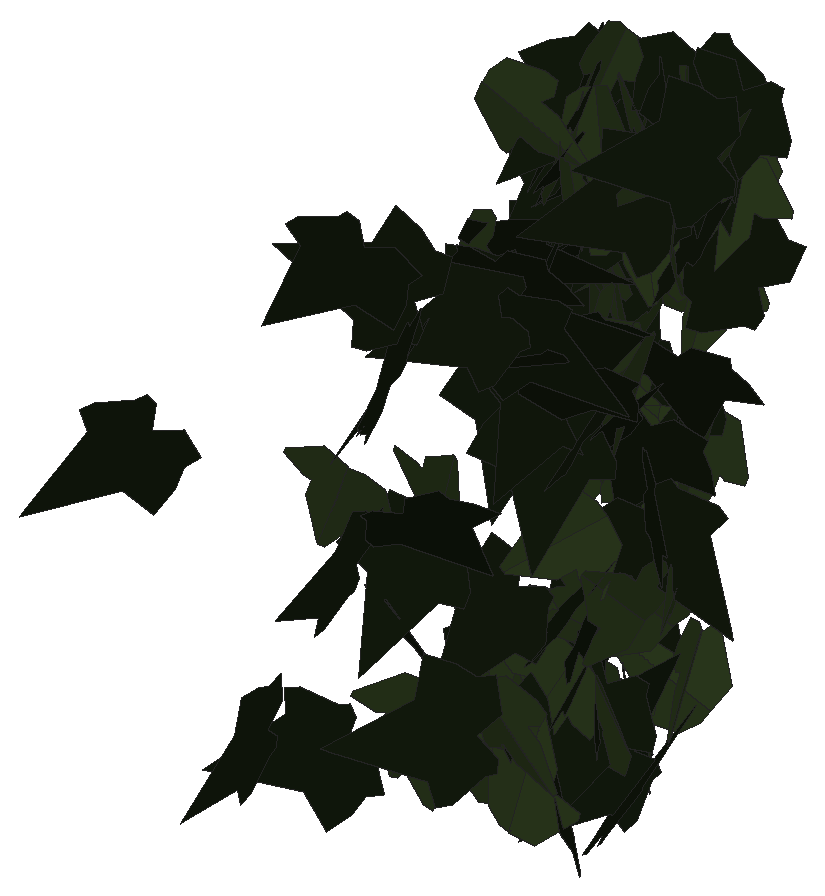
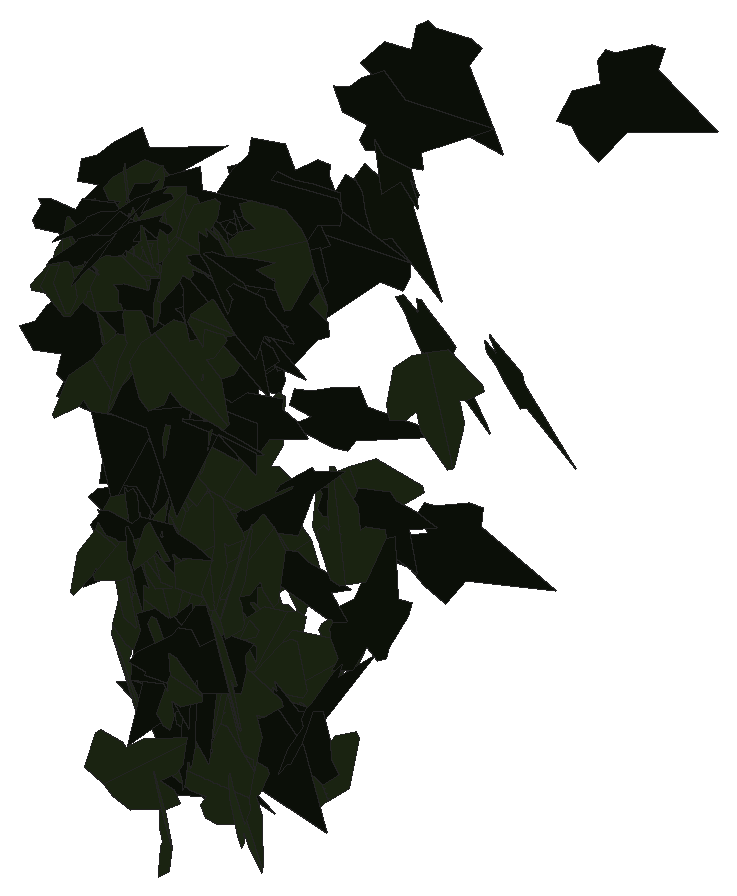
# SketchUp Ruby script. Lengths in inches.
U = 1.inch
M = Sketchup.active_model
def pt(a) = Geom::Point3d.new(a.map { |v| v * U })
def face(e, loops, mat)
  f = e.add_face(loops[0].map { |a| pt(a) })
  loops[1..].each { |l| e.add_face(l.map { |a| pt(a) }).erase! }
  f.material = f.back_material = mat if mat
  f
end
# faces: each face lists its corners as indices into pts; further lists are holes
def faces(e, pts, list, mat = nil) = list.each { |f| face(e, (f[0].is_a?(Array) ? f : [f]).map { |l| l.map { |i| pts[i] } }, mat) }
# xy, xz, yz: faces in a plane at the given z, y or x. An outline is a flat list of corners, or four numbers for a rectangle; further outlines are holes
def ring(l) = l.size == 4 ? [[l[0], l[1]], [l[2], l[1]], [l[2], l[3]], [l[0], l[3]]] : l.each_slice(2).to_a
def flat(e, list, mat, &to3) = list.each { |f| face(e, (f[0].is_a?(Array) ? f : [f]).map { |l| ring(l).map { |u, v| to3.(u, v) } }, mat) }
def xy(e, z, list, mat = nil) = flat(e, list, mat) { |x, y| [x, y, z] }
def xz(e, y, list, mat = nil) = flat(e, list, mat) { |x, z| [x, y, z] }
def yz(e, x, list, mat = nil) = flat(e, list, mat) { |y, z| [x, y, z] }
def lines(e, pts, list) = list.each { |a, b| e.add_line(pt(pts[a]), pt(pts[b])) }
# prism: a flat outline (further loops are holes) pulled along v
def prism(e, loops, v, mat = nil)
  f = face(e, loops, mat); d = Geom::Vector3d.new(v.map { |x| x * U })
  f.pushpull(f.normal.samedirection?(d) ? d.length : -d.length)
end
def box(e, o, s, mat = nil) = prism(e, [[o, [o[0] + s[0], o[1], o[2]], [o[0] + s[0], o[1] + s[1], o[2]], [o[0], o[1] + s[1], o[2]]]], [0, 0, s[2]], mat)
def at(x, y, z, deg = 0) = Geom::Transformation.translation(pt([x, y, z])) * Geom::Transformation.rotation(ORIGIN, Z_AXIS, deg.degrees)
def axes(o, x, y, z) = Geom::Transformation.new([*x, 0, *y, 0, *z, 0, *pt(o).to_a, 1])
def part(name) = M.definitions.add(name)
# library, detail: a bought-in or finely detailed component or shape, given as its bounding box
def library(name, o, s) = part(name).tap { |d| box(d.entities, o, s) }
def detail(e, o, s) = box(e.add_group.entities, o, s)
def put(e, d, t, mat = nil) = e.add_instance(d, t).tap { |i| i.material = mat if mat }
def group(e, t, mat = nil) = e.add_group.tap { |g| g.transformation = t; g.material = mat if mat }.entities
root = M.entities
M.materials.add("efeu1").color = [18, 25, 13]
M.materials.add("efeu2").color = [43, 57, 29]
c1 = part("ivyleaf_9")
p = [[1.54,2.16,1.25],[1.36,2.04,1.19],[-0.21,0.99,0.68],[-0.71,1.11,0.82],[-0.85,0.86,0.67],[-0.8,0.17,0.21],
  [-0.9,-0.01,0.1],[-0.67,-0.16,-0.02],[-0.08,-0.08,-0.05],[-0.03,-0.6,-0.4],[0.65,-0.88,-0.66],[0.83,-0.6,-0.49],
  [1.29,-0.42,-0.43],[1.8125,-0.07,-0.26],[1.21,0.44,0.15]]
faces(c1.entities,p,[[0,1,2,3,4,5,6,7,8,9,10,11,12,13,14]],"efeu1")
c2 = part("ivyleaf_10")
p = [[0,0.5,-0.03],[-0.0625,2.02,-0.43],[-0.19,2.01,-0.46],[-0.54,1.05,-0.29],[-0.52,0.625,-0.18],[-0.83,0.76,-0.28],
  [-1.16,0.64,-0.33],[-1.15,0.33,-0.24],[-0.77,-0.39,0.02],[-0.3,-0.51,0.16],[0.04,-0.48,0.23],[-0.02,2.01,-0.4375],
  [-0.06,2.01,-0.43],[0.04,-0.49,0.23],[0.67,-0.49,0.14],[1.38,0.36,-0.2],[1.375,0.51,-0.24],[0.81,0.65,-0.19],
  [0.62,0.59,-0.15],[0.6,1.09,-0.28],[0.5,1.23,-0.31]]
faces(c2.entities,p,[[0,1,2,3,4,5,6,7,8,9,10],[11,12,0,13,14,15,16,17,18,19,20]],"efeu2")
put(root,c1,axes([51.93,217.2,212.98],[-0.05869,0.02643,-0.49584],[-0.02771,-0.49869,-0.02331],[-0.49577,0.02474,0.06]))
put(root,c1,axes([52.75,217.98,209.62],[-0.43052,0.24134,-0.08007],[0.06799,-0.04247,-0.49353],[-0.24502,-0.43584,0.00375]))
put(root,c1,axes([53.94,219.7,209.25],[-0.36119,-0.02977,0.34447],[-0.33695,-0.08134,-0.36034],[0.0775,-0.49244,0.0387]))
put(root,c1,axes([52.6875,219.4375,210.8],[-0.36273,0.34249,0.03353],[-0.02659,0.02067,-0.49886],[-0.3431,-0.36369,0.00322]))
put(root,c1,axes([52.63,219.63,214.2],[0.07664,0.12487,-0.47805],[-0.2722,-0.39307,-0.14631],[-0.41235,0.28268,0.00773]))
put(root,c1,axes([53.43,219.36,211.66],[0.38543,0.31697,0.03117],[0.02393,0.01998,-0.49903],[-0.3176,0.38617,0.00023]))
put(root,c1,axes([52.1875,219.87,208.45],[-0.09347,-0.05912,-0.48761],[-0.29492,-0.39018,0.10384],[-0.39279,0.30703,0.03807]))
put(root,c1,axes([53.15,219.4375,213],[-0.26005,0.14295,-0.40242],[-0.35072,0.19733,0.29674],[0.24366,0.43661,-0.00237]))
put(root,c1,axes([52.75,220.04,212.73],[-0.3149,0.36073,-0.14391],[0.09485,-0.10823,-0.47884],[-0.37662,-0.32887,-0.00026]))
put(root,c1,axes([52.8,220.15,213.5],[-0.19213,0.03222,0.46049],[-0.45006,0.09779,-0.19462],[-0.10261,-0.48928,-0.00858]))
put(root,c2,axes([52.88,220.35,208.99],[-0.34204,-0.31812,0.17834],[-0.12668,-0.12564,-0.46708],[0.34199,-0.36471,0.00535]))
put(root,c2,axes([51.69,220.57,210.91],[-0.44087,-0.09357,0.21651],[-0.21259,-0.04117,-0.45068],[0.10217,-0.48944,-0.00348]))
put(root,c1,axes([53.06,221.26,212.93],[-0.44488,0.00063,0.22821],[-0.2282,0.0041,-0.44487],[-0.00243,-0.49998,-0.00336]))
put(root,c2,axes([53.04,221.24,208.59],[-0.34431,0.11872,-0.34257],[0.31834,-0.12712,-0.36401],[-0.17352,-0.46877,0.01195]))
put(root,c2,axes([53.32,221.22,207.57],[0.49184,-0.06443,-0.06276],[0.06362,0.00252,0.49593],[-0.06359,-0.49582,0.01068]))
put(root,c1,axes([53.13,221.28,212.82],[-0.00254,0.00286,-0.49999],[0.32697,0.37827,0.0005],[0.37827,-0.32696,-0.00379]))
put(root,c1,axes([51.81,221.65,209.79],[-0.43015,-0.23233,-0.10487],[0.09824,0.03872,-0.48872],[0.23521,-0.44105,0.01234]))
put(root,c1,axes([53.32,221.89,207.32],[0.01934,-0.13736,0.48037],[0.09828,-0.47029,-0.13844],[0.48986,0.09978,0.00881]))
put(root,c2,axes([52.15,221.25,207.87],[-0.05823,0.33651,0.3652],[-0.08192,0.35616,-0.34124],[-0.48979,-0.09957,0.01365]))
put(root,c1,axes([52.92,221.4,213.36],[0.37757,0.25861,-0.2014],[-0.16846,-0.11045,-0.45763],[-0.28118,0.41343,0.00373]))
put(root,c1,axes([53.12,221.95,211.875],[-0.13061,-0.44021,0.19788],[-0.03696,-0.19528,-0.4588],[0.48122,-0.13448,0.01847]))
put(root,c1,axes([53.29,221.82,211.52],[-0.196,-0.45231,-0.08365],[0.02284,0.08124,-0.49283],[0.45941,-0.19701,-0.01119]))
put(root,c1,axes([53.73,221.59,212.36],[0.10603,0.32943,-0.36088],[-0.27049,-0.26797,-0.32408],[-0.40693,0.26395,0.12139]))
put(root,c1,axes([51.4,221.99,208.34],[0.42363,-0.26443,-0.02474],[0.03192,0.00445,0.49896],[-0.26366,-0.42433,0.02065]))
put(root,c1,axes([53.04,222.08,212.15],[0.02976,-0.02806,0.49832],[0.40241,-0.29397,-0.04059],[0.29527,0.40348,0.00508]))
put(root,c1,axes([53.57,221.85,211.4375],[-0.20148,0.4259,0.16738],[-0.10421,0.13538,-0.46991],[-0.44559,-0.22424,0.03421]))
put(root,c2,axes([51.84,222.36,212.6875],[-0.0193,-0.03197,-0.4986],[0.33338,-0.37248,0.01098],[-0.37214,-0.33202,0.03569]))
put(root,c1,axes([52.36,222.34,209.14],[-0.47848,-0.13346,-0.05695],[0.05755,0.0056,-0.49665],[0.1332,-0.48183,0.01]))
put(root,c2,axes([51.3,222.49,209.61],[-0.43722,0.08105,0.22863],[0.22455,-0.04302,0.44467],[0.09175,0.49151,0.00123]))
put(root,c1,axes([51.55,222.87,207.64],[0.14864,-0.28493,-0.38304],[0.22933,-0.30924,0.31902],[-0.41871,-0.27053,0.03876]))
put(root,c2,axes([52.8125,222.51,208.34],[0.45497,-0.06468,-0.19703],[-0.19487,0.0291,-0.45954],[0.07091,0.49494,0.00128]))
put(root,c1,axes([52.34,222.53,212.04],[-0.03092,0.36078,0.3448],[0.01889,-0.34436,0.36202],[0.49869,0.03542,0.00767]))
put(root,c2,axes([51.55,222.59,206.85],[-0.38038,-0.0109,0.32433],[0.32434,0.00379,0.38051],[-0.01075,0.49987,0.00419]))
put(root,c2,axes([51.94,222.21,207.86],[0.0691,0.11293,0.48215],[0.08248,0.4774,-0.12363],[-0.48829,0.09662,0.04734]))
put(root,c2,axes([52.95,222.68,209.9],[0.32792,0.01853,-0.377],[-0.37564,-0.03294,-0.32835],[-0.037,0.49857,-0.00768]))
put(root,c1,axes([53.07,222.39,209.17],[-0.17356,0.45442,0.11566],[-0.06062,0.10055,-0.48602],[-0.46498,-0.18273,0.02019]))
put(root,c1,axes([53.4,222.24,211.17],[0.10808,0.41603,0.25542],[0.02456,0.25664,-0.42841],[-0.48756,0.10515,0.03504]))
put(root,c1,axes([52.91,222.76,208.43],[-0.36094,0.22076,-0.26643],[0.21911,-0.15213,-0.4229],[-0.26778,-0.42204,0.01308]))
put(root,c1,axes([52.98,222.96,208],[-0.24907,-0.4328,0.02543],[0.01012,-0.03513,-0.49866],[0.43343,-0.24788,0.02626]))
put(root,c2,axes([53.52,222.47,207.88],[-0.14103,0.1618,-0.45159],[-0.32263,0.31634,0.2141],[0.35499,0.35178,0.01518]))
put(root,c1,axes([51.7,222.76,207.06],[-0.14899,0.10833,0.46483],[0.32585,-0.33272,0.18198],[0.34874,0.35716,0.02854]))
put(root,c2,axes([53.14,223.1,211.6],[-0.00318,-0.08574,0.49258],[0.13006,-0.47578,-0.08197],[0.48278,0.12761,0.02533]))
put(root,c2,axes([53.3125,223.04,208.92],[-0.12369,-0.31974,-0.36396],[-0.14542,-0.33381,0.34267],[-0.46212,0.19063,-0.01042]))
put(root,c1,axes([51.87,222.54,212.63],[0.37549,0.06671,0.32335],[0.31648,0.06677,-0.38129],[-0.09405,0.49101,0.00792]))
put(root,c1,axes([53.41,222.49,206.82],[-0.19352,0.45369,-0.08194],[-0.03315,0.07495,0.49324],[0.45984,0.19633,0.00108]))
put(root,c1,axes([52.7,222.59,211.97],[0.33303,0.3726,-0.01596],[-0.01069,-0.01185,-0.49975],[-0.37279,0.33321,0.00007]))
put(root,c1,axes([52.32,222.85,207.35],[0.02988,0.23247,-0.44166],[-0.37496,-0.28157,-0.17357],[-0.32942,0.34158,0.1575]))
put(root,c2,axes([52.15,222.67,208.53],[0.09058,0.43775,0.22398],[0.02329,0.22367,-0.44657],[-0.49117,0.09134,0.02013]))
put(root,c1,axes([53.49,223.2,213.49],[-0.2892,-0.17302,0.36936],[-0.32093,-0.18292,-0.33697],[0.25173,-0.43198,-0.00525]))
put(root,c2,axes([52.75,223.1875,211.74],[0.07905,-0.10737,-0.4819],[0.26888,-0.39995,0.13322],[-0.41407,-0.28021,-0.0055]))
put(root,c2,axes([53.3125,223.13,211.71],[0.22234,-0.40073,0.19996],[0.09517,-0.17586,-0.45827],[0.43761,0.24185,-0.00193]))
put(root,c2,axes([52.22,222.8,208.28],[-0.21629,-0.35255,-0.28094],[0.14733,0.23921,-0.41361],[0.42604,-0.2617,0.0004]))
put(root,c1,axes([52.91,222.82,208],[0.08149,-0.0056,-0.49328],[-0.48911,0.06421,-0.08153],[0.06426,0.49583,0.00499]))
put(root,c1,axes([53.07,223.23,207.19],[-0.49847,0.0167,0.03535],[-0.03569,-0.01007,-0.49862],[-0.01595,-0.49962,0.01123]))
put(root,c1,axes([52.95,222.9,207.4375],[-0.22353,0.43739,0.09344],[-0.04941,0.07967,-0.49113],[-0.44452,-0.2288,0.00761]))
put(root,c2,axes([52.8125,223.22,208.75],[-0.4478,-0.04873,-0.21704],[-0.21272,-0.0488,0.44985],[-0.06502,0.49522,0.02297]))
put(root,c1,axes([51.56,223.46,210.69],[-0.11731,-0.48455,0.03803],[-0.00547,-0.0378,-0.49854],[0.48601,-0.11738,0.00356]))
put(root,c1,axes([52.84,222.8125,208.25],[0.03725,0.03445,0.49742],[0.17231,0.46719,-0.04526],[-0.46789,0.17479,0.02294]))
put(root,c1,axes([53.81,223.58,213.92],[-0.21312,-0.12866,0.43362],[-0.34871,-0.25855,-0.2481],[0.28807,-0.40816,0.02047]))
put(root,c1,axes([53.43,223.1,210.26],[0.23797,-0.09851,-0.42856],[-0.39489,0.16652,-0.25755],[0.19347,0.46105,0.00145]))
put(root,c2,axes([52.35,223.31,207.93],[-0.43351,-0.13752,0.20775],[-0.19934,-0.05864,-0.45478],[0.14945,-0.47713,-0.00399]))
put(root,c1,axes([53.28,223.31,210.83],[0.25711,0.20304,-0.37771],[-0.28476,-0.24845,-0.32739],[-0.32064,0.38346,-0.01212]))
put(root,c2,axes([53.13,223.62,208.57],[-0.23156,-0.26907,-0.35211],[-0.2427,-0.2554,0.35478],[-0.37078,0.33522,-0.01232]))
put(root,c2,axes([51.45,223.36,213.87],[-0.24625,0.0433,-0.433],[0.42583,-0.07849,-0.25002],[-0.08962,-0.4919,0.00178]))
put(root,c1,axes([53.29,223.29,209.88],[-0.11782,-0.18414,-0.44968],[0.24248,0.37871,-0.2186],[0.4211,-0.26958,0.00006]))
put(root,c1,axes([52.46,223.21,206.98],[-0.04662,-0.14522,0.47617],[0.46851,0.14888,0.09128],[-0.16829,0.45469,0.12219]))
put(root,c2,axes([53.43,223.18,213.75],[-0.18692,-0.25812,-0.38527],[0.21897,0.31705,-0.31865],[0.4088,-0.28784,-0.00548]))
put(root,c2,axes([53.68,223.18,213.02],[-0.03548,0.02569,0.49808],[-0.41201,0.27987,-0.04378],[-0.28104,-0.41354,0.00131]))
put(root,c2,axes([53.3,223.82,209.26],[0.07977,-0.12907,0.47642],[0.29408,-0.37517,-0.15088],[0.39642,0.30429,0.01606]))
put(root,c2,axes([53.04,223.45,213.18],[0.29978,0.39559,0.06035],[0.03471,0.04941,-0.49634],[-0.39866,0.30177,0.00217]))
put(root,c2,axes([51.7,223.51,210.15],[-0.41829,0.14489,-0.23246],[0.2161,-0.08617,-0.44258],[-0.16832,-0.47072,0.00947]))
put(root,c2,axes([52.72,223.83,211.36],[0.02205,-0.32082,-0.38287],[0.11483,-0.36972,0.31642],[-0.48614,-0.10188,0.05737]))
put(root,c2,axes([52.29,223.64,213.84],[0.42049,-0.13497,0.23446],[0.2362,-0.02811,-0.43979],[0.1319,0.48062,0.04012]))
put(root,c2,axes([53.45,223.71,208.24],[0.31321,-0.38603,0.05366],[0.03384,-0.04164,-0.49711],[0.38827,0.31503,0.00005]))
put(root,c1,axes([53.53,223.45,211.62],[0.35215,0.26501,-0.23614],[-0.19765,-0.1299,-0.44052],[-0.29483,0.40361,0.01327]))
put(root,c1,axes([52.0625,223.86,213],[-0.47016,-0.1664,0.03554],[-0.02789,-0.02768,-0.49845],[0.16786,-0.47068,0.01675]))
put(root,c1,axes([53.76,223.29,212.92],[-0.32596,0.29399,-0.23942],[-0.17355,0.16502,0.43892],[0.33709,0.36924,-0.00554]))
put(root,c2,axes([52.05,223.625,213.32],[-0.15688,0.4703,-0.06488],[0.00927,-0.06528,-0.49563],[-0.47466,-0.15671,0.01176]))
put(root,c2,axes([53.19,223.53,213.5625],[-0.28541,0.23891,-0.33386],[-0.26779,0.19986,0.37194],[0.31117,0.39112,0.01387]))
put(root,c2,axes([51.73,223.91,211.13],[-0.25426,-0.30277,-0.30607],[-0.19788,-0.2335,0.39537],[-0.38235,0.32219,-0.00108]))
put(root,c2,axes([52.67,224,213.42],[-0.04976,0.146,-0.47561],[0.08246,-0.46895,-0.15258],[-0.49064,-0.09363,0.02259]))
put(root,c2,axes([51.73,223.8,207.15],[0.19585,-0.45436,0.07211],[0.02885,-0.06609,-0.49477],[0.45914,0.19796,0.00033]))
put(root,c2,axes([52.19,224.07,210.08],[-0.03056,-0.03225,-0.49802],[-0.24978,-0.43098,0.04324],[-0.43206,0.25143,0.01023]))
put(root,c1,axes([52.41,224.02,210.47],[-0.08721,0.18911,0.45457],[-0.15716,-0.44819,0.1563],[0.46658,-0.11562,0.13762]))
put(root,c1,axes([52.08,223.81,213.4375],[-0.22126,0.40258,-0.19742],[0.08349,-0.17931,-0.45922],[-0.44054,-0.23618,0.01213]))
put(root,c2,axes([52.47,224.17,210.01],[-0.0688,0.13984,0.47509],[-0.0419,-0.47958,0.13509],[0.49347,-0.02122,0.07771]))
put(root,c2,axes([52.32,223.78,210.36],[-0.45833,0.01768,0.19904],[-0.19948,-0.01109,-0.45835],[-0.01179,-0.49956,0.01722]))
put(root,c1,axes([52.69,224.11,213.16],[-0.44125,-0.23327,-0.02967],[0.0307,0.00539,-0.49903],[0.23314,-0.44221,0.00957]))
put(root,c1,axes([52.55,223.79,208.85],[-0.07089,0.47495,-0.13927],[0.03552,-0.13544,-0.47999],[-0.49367,-0.07795,-0.01453]))
put(root,c1,axes([52,224.23,213.83],[-0.43338,-0.23137,0.09302],[-0.0267,-0.14238,-0.47855],[0.24793,-0.41976,0.11106]))
put(root,c1,axes([51.95,224.03,214.02],[-0.37445,0.20765,-0.25821],[0.22109,-0.13364,-0.42809],[-0.2468,-0.43477,0.00826]))
put(root,c1,axes([51.64,224.05,212.1],[-0.29182,-0.32475,-0.24369],[0.16106,0.18288,-0.43659],[0.3727,-0.33331,-0.00213]))
put(root,c2,axes([51.78,223.88,207.2],[-0.05507,-0.01212,0.49681],[0.47605,0.14219,0.05624],[-0.14265,0.4792,-0.00412]))
put(root,c2,axes([52.99,224.1,214.12],[0.35088,-0.26559,0.23738],[0.21192,-0.11218,-0.43875],[0.28632,0.40851,0.03384]))
put(root,c1,axes([52.03,223.95,212.63],[0.06959,0.38585,-0.31029],[-0.0951,-0.29709,-0.39076],[-0.48592,0.1134,0.03204]))
put(root,c2,axes([52.09,224.04,211.93],[-0.33755,0.26752,-0.25396],[0.17683,-0.18475,-0.42965],[-0.32372,-0.37987,0.03011]))
put(root,c1,axes([52.17,224.21,211.65],[-0.44563,-0.21604,-0.06881],[0.06983,0.01359,-0.49491],[0.21572,-0.45071,0.01806]))
put(root,c2,axes([52.31,223.99,211.78],[-0.30185,0.39083,-0.07837],[-0.00064,-0.09878,-0.49015],[-0.39861,-0.2958,0.06013]))
put(root,c2,axes([51.82,224.03,209.1],[0.31968,-0.37431,-0.08772],[-0.04826,0.07411,-0.49212],[0.38141,0.32311,0.01126]))
put(root,c1,axes([51.63,224.18,213.55],[-0.39142,-0.17996,-0.25379],[0.23026,0.10673,-0.4308],[0.20922,-0.45412,-0.00067]))
put(root,c2,axes([52.02,224.35,211.26],[0.00985,-0.35846,-0.34844],[0.00216,-0.34847,0.35856],[-0.4999,-0.00857,-0.00532]))
put(root,c2,axes([51.8,223.8,212.8],[0.10525,-0.3053,0.38173],[-0.11377,0.36445,0.32285],[-0.47537,-0.15482,0.00724]))
put(root,c1,axes([52.02,224.36,207.77],[0.02329,-0.03772,0.49803],[0.08558,-0.4909,-0.04118],[0.49207,0.08716,-0.01641]))
put(root,c2,axes([52.05,224.34,214.13],[0.04424,0.34618,-0.35806],[-0.087,-0.34857,-0.34775],[-0.49038,0.09307,0.02939]))
put(root,c1,axes([53.01,224.41,213.88],[0.0499,-0.48157,0.12489],[0.01506,-0.12399,-0.48415],[0.49728,0.05208,0.00212]))
put(root,c1,axes([53.74,224.3125,212.16],[-0.08323,0.01937,0.49264],[-0.48982,-0.06011,-0.08038],[0.05611,-0.496,0.02899]))
put(root,c1,axes([52.13,224.04,208.87],[-0.01712,-0.28728,-0.40887],[0.02956,0.40781,-0.28777],[0.49883,-0.03403,0.00302]))
put(root,c2,axes([53.52,224.49,213.55],[-0.03544,0.2032,-0.45547],[-0.1072,-0.44905,-0.192],[-0.48709,0.08404,0.07539]))
put(root,c2,axes([52.23,224.49,206.75],[0.01841,-0.03538,-0.49841],[0.25038,-0.43096,0.03984],[-0.4324,-0.25105,0.00185]))
put(root,c2,axes([53.27,224.36,212.15],[0.14651,0.41234,-0.24188],[-0.07365,-0.2305,-0.43754],[-0.47235,0.16384,-0.0068]))
put(root,c2,axes([52.27,224.38,210.67],[0.05205,0.42331,-0.26096],[-0.06409,-0.25449,-0.42559],[-0.49314,0.07775,0.02777]))
put(root,c2,axes([53.51,224.51,213.42],[0.13805,0.11357,-0.46695],[-0.33773,-0.3227,-0.17833],[-0.34188,0.36465,-0.01238]))
put(root,c2,axes([51.55,224.19,209.75],[-0.31999,0.37364,-0.08942],[-0.05769,0.06833,0.49194],[0.37984,0.32515,-0.00062]))
put(root,c2,axes([52.54,224.3,210.1],[0.33011,0.36265,-0.09754],[-0.06588,-0.07194,-0.49039],[-0.36971,0.33662,0.00029]))
put(root,c2,axes([53.43,224.31,213.25],[0.43447,0.23963,-0.06175],[-0.06056,-0.01801,-0.49599],[-0.23993,0.43847,0.01338]))
put(root,c1,axes([53.44,224.49,214.07],[-0.39918,-0.26839,-0.13647],[0.11329,0.07608,-0.48102],[0.27896,-0.41495,0.00007]))
put(root,c2,axes([53.1,224.51,210.1875],[0.04001,0.36658,-0.33767],[-0.07036,-0.3312,-0.3679],[-0.4934,0.07696,0.02508]))
put(root,c1,axes([52.7,224.49,210.39],[-0.25153,0.115,-0.41654],[0.3828,-0.16432,-0.27652],[-0.2005,-0.45801,-0.00538]))
put(root,c2,axes([52.6,224.19,208.53],[0.0937,-0.02233,0.49063],[-0.48429,0.07894,0.09608],[-0.08175,-0.49322,-0.00684]))
put(root,c2,axes([52.99,223.98,212.31],[-0.03164,0.08124,0.49234],[-0.25726,0.42006,-0.08585],[-0.42757,-0.25875,0.01522]))
put(root,c1,axes([52.91,224.5,214.28],[0.01778,-0.48729,-0.1106],[0.11171,0.11174,-0.47438],[0.48704,-0.00784,0.11285]))
put(root,c1,axes([52.21,224.13,212.2],[0.20677,0.43948,-0.11875],[-0.1272,-0.06945,-0.47854],[-0.43711,0.2281,0.08308]))
put(root,c2,axes([52.83,224.48,207.23],[0.23058,0.22082,0.3848],[-0.2965,-0.2459,0.31878],[0.33003,-0.3752,0.01755]))
put(root,c1,axes([52.96,224.54,213.96],[-0.04372,-0.47991,-0.13333],[0.10512,0.12194,-0.47337],[0.48686,-0.06943,0.09023]))
put(root,c1,axes([52.51,224.65,210.55],[-0.39527,-0.25237,-0.17341],[0.17673,0.0432,-0.46572],[0.25005,-0.42947,0.05505]))
put(root,c2,axes([52.13,224.57,212.8],[-0.31306,-0.17431,0.34872],[-0.28499,-0.20286,-0.35725],[0.26603,-0.42245,0.02767]))
